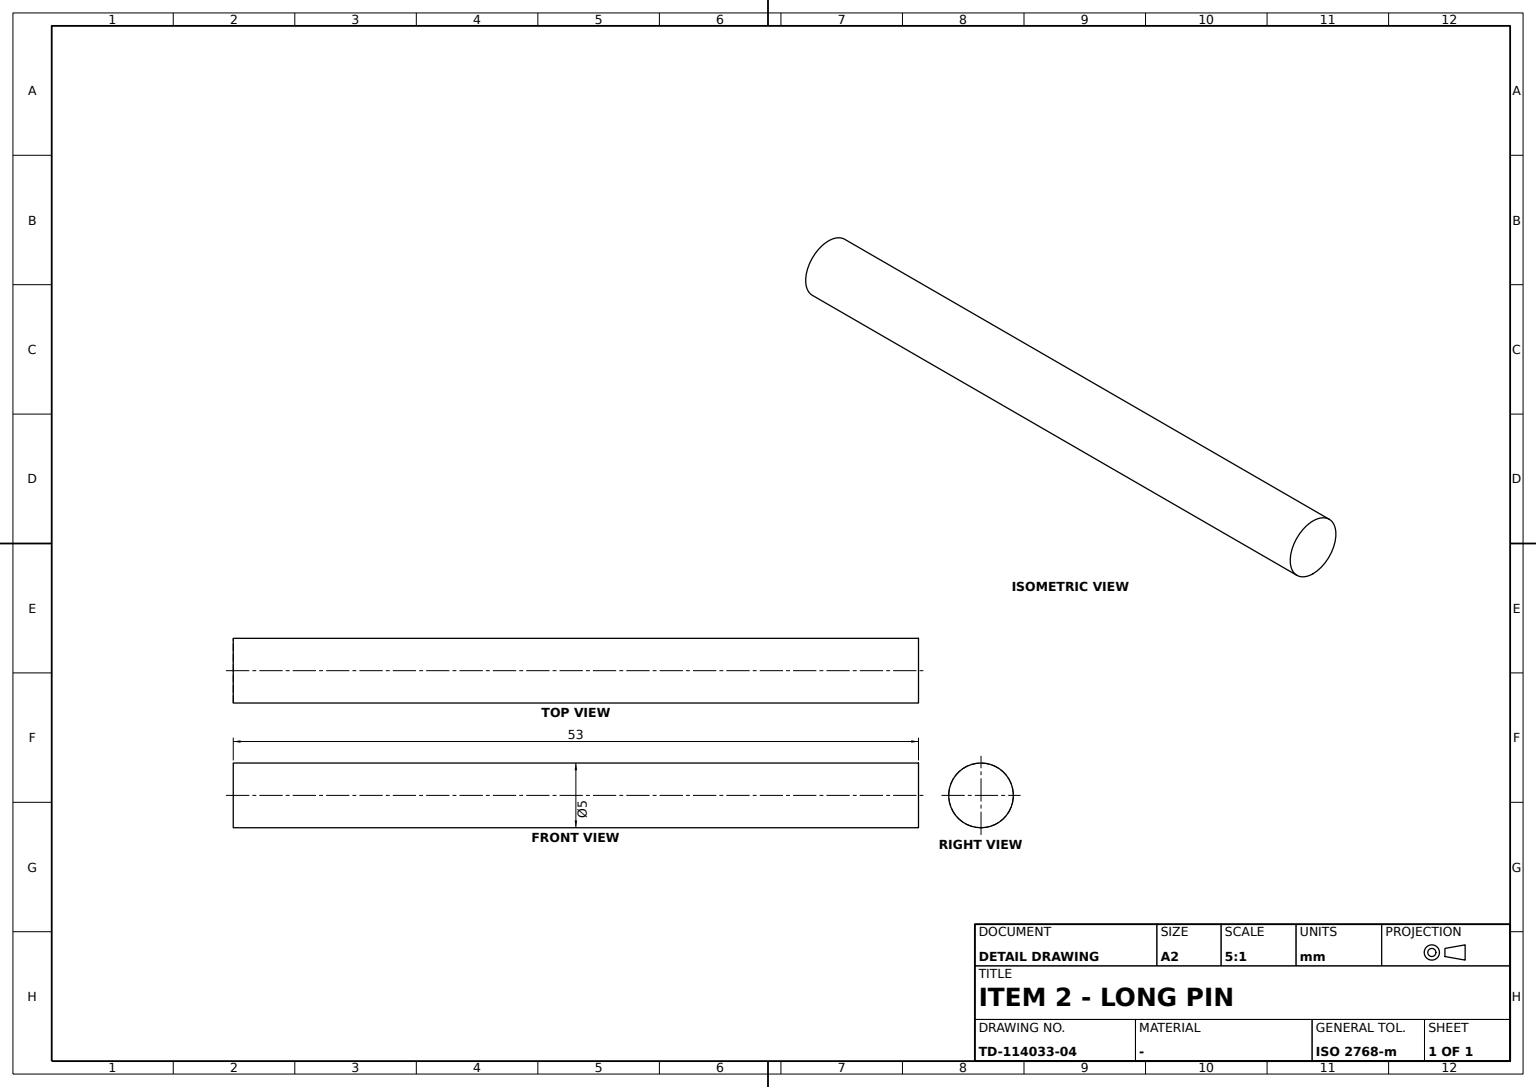
ISO-10303-21;
HEADER;
FILE_DESCRIPTION((''),'2;1');
FILE_NAME('','',(''),(''),'','','');
FILE_SCHEMA(('AUTOMOTIVE_DESIGN'));
ENDSEC;
DATA;
#1=APPLICATION_CONTEXT('');
#2=PRODUCT_CONTEXT('',#1,'mechanical');
#3=PRODUCT('','','',(#2));
#4=PRODUCT_DEFINITION_FORMATION('','',#3);
#5=PRODUCT_DEFINITION_CONTEXT('',#1,'design');
#6=PRODUCT_DEFINITION('','',#4,#5);
#7=PRODUCT_DEFINITION_SHAPE('','',#6);
#8=(LENGTH_UNIT()NAMED_UNIT(*)SI_UNIT(.MILLI.,.METRE.));
#9=(NAMED_UNIT(*)PLANE_ANGLE_UNIT()SI_UNIT($,.RADIAN.));
#10=(NAMED_UNIT(*)SI_UNIT($,.STERADIAN.)SOLID_ANGLE_UNIT());
#11=UNCERTAINTY_MEASURE_WITH_UNIT(LENGTH_MEASURE(0.005),#8,'distance_accuracy_value','');
#12=(GEOMETRIC_REPRESENTATION_CONTEXT(3)GLOBAL_UNCERTAINTY_ASSIGNED_CONTEXT((#11))GLOBAL_UNIT_ASSIGNED_CONTEXT((#8,#9,#10))REPRESENTATION_CONTEXT('',''));
#13=CARTESIAN_POINT('',(-26.5,0.,-2.5));
#14=VERTEX_POINT('',#13);
#15=CARTESIAN_POINT('',(-26.5,0.,0.));
#16=DIRECTION('',(1.,0.,0.));
#17=DIRECTION('',(0.,0.,-1.));
#18=AXIS2_PLACEMENT_3D('',#15,#16,#17);
#19=CIRCLE('',#18,2.5);
#20=EDGE_CURVE('',#14,#14,#19,.T.);
#21=ORIENTED_EDGE('',*,*,#20,.F.);
#22=EDGE_LOOP('',(#21));
#23=FACE_BOUND('',#22,.T.);
#24=DIRECTION('',(0.,1.,0.));
#25=AXIS2_PLACEMENT_3D('',#15,#16,#24);
#26=PLANE('',#25);
#27=ADVANCED_FACE('',(#23),#26,.F.);
#28=CARTESIAN_POINT('',(26.5,0.,-2.5));
#29=VERTEX_POINT('',#28);
#30=CARTESIAN_POINT('',(26.5,0.,0.));
#31=AXIS2_PLACEMENT_3D('',#30,#16,#17);
#32=CIRCLE('',#31,2.5);
#33=EDGE_CURVE('',#29,#29,#32,.T.);
#34=ORIENTED_EDGE('',*,*,#33,.T.);
#35=EDGE_LOOP('',(#34));
#36=FACE_BOUND('',#35,.T.);
#37=AXIS2_PLACEMENT_3D('',#30,#16,#24);
#38=PLANE('',#37);
#39=ADVANCED_FACE('',(#36),#38,.T.);
#40=ORIENTED_EDGE('',*,*,#33,.F.);
#41=EDGE_LOOP('',(#40));
#42=FACE_BOUND('',#41,.T.);
#43=ORIENTED_EDGE('',*,*,#20,.T.);
#44=EDGE_LOOP('',(#43));
#45=FACE_BOUND('',#44,.T.);
#46=CARTESIAN_POINT('',(0.,0.,0.));
#47=AXIS2_PLACEMENT_3D('',#46,#16,#24);
#48=CYLINDRICAL_SURFACE('',#47,2.5);
#49=ADVANCED_FACE('',(#42,#45),#48,.T.);
#50=CLOSED_SHELL('',(#27,#39,#49));
#51=MANIFOLD_SOLID_BREP('',#50);
#52=ADVANCED_BREP_SHAPE_REPRESENTATION('',(#51),#12);
#53=SHAPE_DEFINITION_REPRESENTATION(#7,#52);
ENDSEC;
END-ISO-10303-21;
